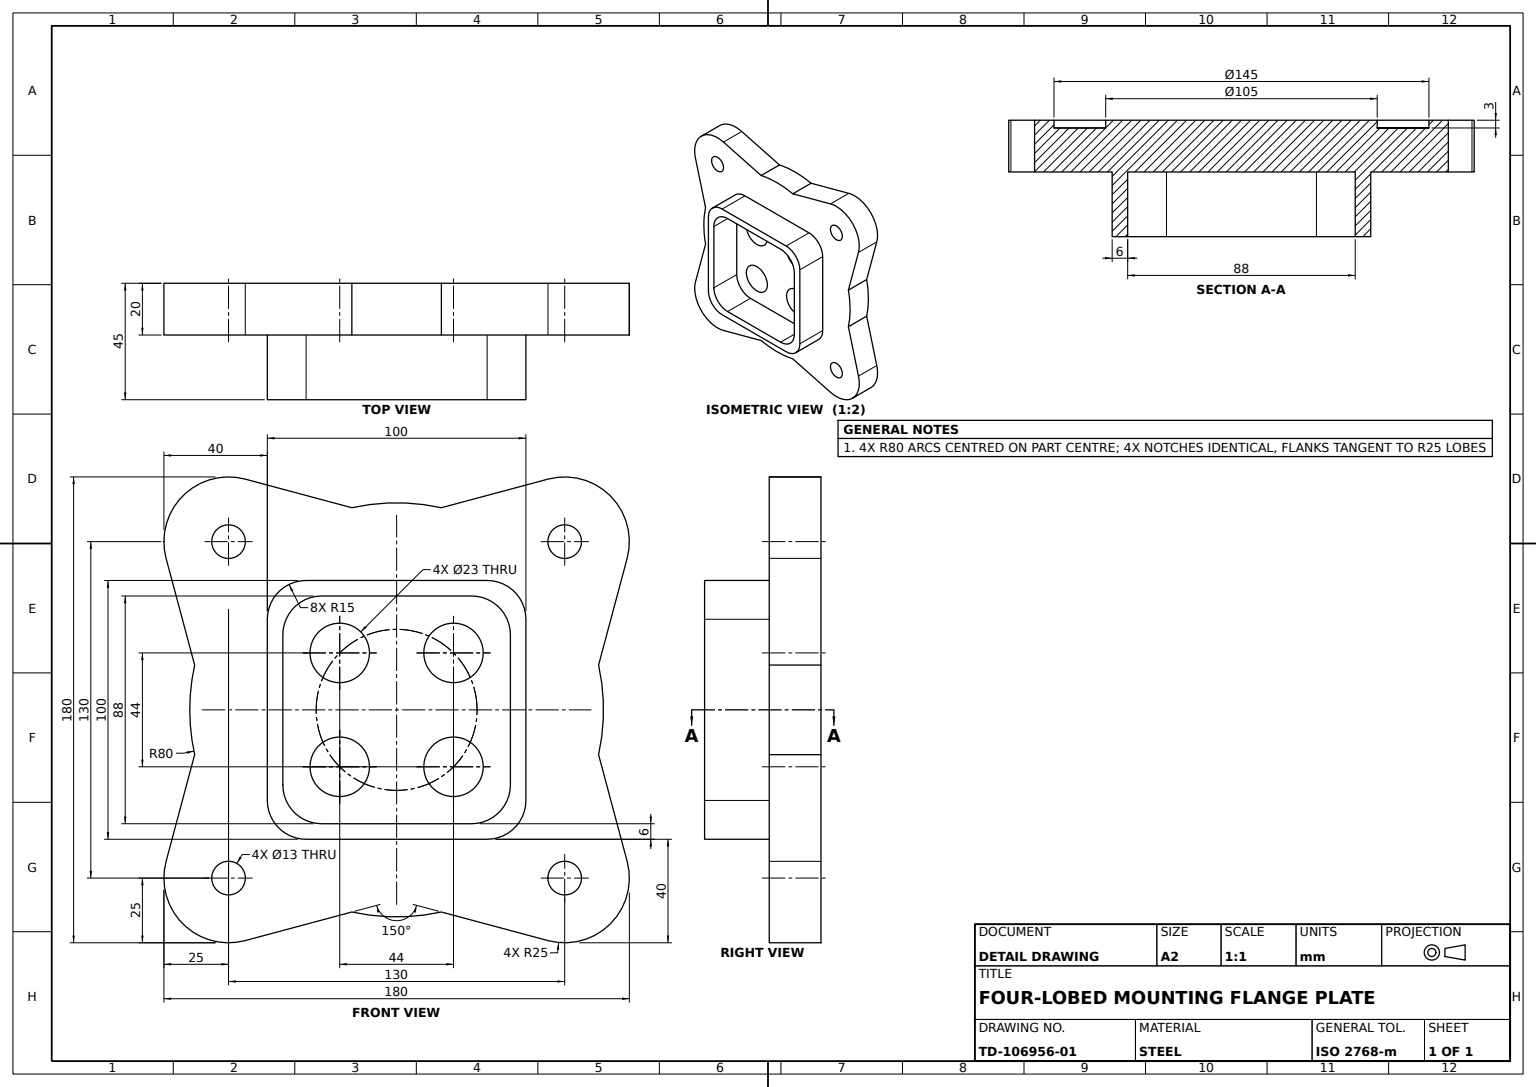
solid
v1 (89.148146,-58.529524,20)
v2 (89.148146,-58.529524,0)
e1 v1 v2 LINE
v3 (78.104184,-17.312898,0)
e2 v2 v3 LINE
v4 (78.104184,-17.312898,20)
e3 v4 v3 LINE
e4 v1 v4 LINE
face PLANE(AX(P(68.543971,18.366302,20),D(-0.965925826,-0.258819045,0),D(0.258819045,-0.965925826,0))) rev [e1 e2 -e3 -e4]
v5 (52.5,0,3)
v6 (-52.5,0,3)
e5 v5 v6 CIRCLE(AX(P(0,0,3),D(0,0,-1),D(-1,0,0)),52.5)
v7 (-52.5,0,0)
e6 v6 v7 LINE
v8 (52.5,0,0)
e7 v8 v7 CIRCLE(AX(P(0,0,0),D(0,0,-1),D(-1,0,0)),52.5)
e8 v5 v8 LINE
face CYL(AX(P(0,0,3),D(0,0,-1),D(-1,0,0)),52.5) [e5 e6 -e7 -e8]
v9 (-50,35,45)
v10 (-35,50,45)
e9 v9 v10 CIRCLE(AX(P(-35,35,45),D(0,0,-1),D(1,0,0)),15)
v11 (-35,50,20)
e10 v10 v11 LINE
v12 (-50,35,20)
e11 v12 v11 CIRCLE(AX(P(-35,35,20),D(0,0,-1),D(1,0,0)),15)
e12 v9 v12 LINE
face CYL(AX(P(-35,35,45),D(0,0,-1),D(-1,0,0)),15) [e9 e10 -e11 -e12]
e13 v6 v5 CIRCLE(AX(P(0,0,3),D(0,0,-1),D(-1,0,0)),52.5)
v13 (-72.5,0,3)
v14 (72.5,0,3)
e14 v13 v14 CIRCLE(AX(P(0,0,3),D(0,0,-1),D(-1,0,0)),72.5)
e15 v14 v13 CIRCLE(AX(P(0,0,3),D(0,0,-1),D(-1,0,0)),72.5)
face PLANE(AX(P(0,0,3),D(0,0,-1),D(-1,0,0))) [-e5 -e13] [e14 e15]
v15 (-50,-35,45)
e16 v15 v9 LINE
v16 (-35,-50,45)
e17 v15 v16 CIRCLE(AX(P(-35,-35,45),D(0,0,1),D(1,0,0)),15)
v17 (35,-50,45)
e18 v16 v17 LINE
v18 (50,-35,45)
e19 v17 v18 CIRCLE(AX(P(35,-35,45),D(0,0,1),D(1,0,0)),15)
v19 (50,35,45)
e20 v18 v19 LINE
v20 (35,50,45)
e21 v19 v20 CIRCLE(AX(P(35,35,45),D(0,0,1),D(1,0,0)),15)
e22 v10 v20 LINE
v21 (-29,44,45)
v22 (29,44,45)
e23 v21 v22 LINE
v23 (44,29,45)
e24 v23 v22 CIRCLE(AX(P(29,29,45),D(0,0,1),D(1,0,0)),15)
v24 (44,-29,45)
e25 v24 v23 LINE
v25 (29,-44,45)
e26 v25 v24 CIRCLE(AX(P(29,-29,45),D(0,0,1),D(1,0,0)),15)
v26 (-29,-44,45)
e27 v26 v25 LINE
v27 (-44,-29,45)
e28 v26 v27 CIRCLE(AX(P(-29,-29,45),D(0,0,-1),D(1,0,0)),15)
v28 (-44,29,45)
e29 v27 v28 LINE
e30 v28 v21 CIRCLE(AX(P(-29,29,45),D(0,0,-1),D(1,0,0)),15)
face PLANE(AX(P(0,0,45),D(0,0,1),D(1,0,0))) [-e9 -e16 e17 e18 e19 e20 e21 -e22] [e23 -e24 -e25 -e26 -e27 e28 e29 e30]
v29 (-35,-50,20)
e31 v16 v29 LINE
v30 (-50,-35,20)
e32 v15 v30 LINE
e33 v30 v29 CIRCLE(AX(P(-35,-35,20),D(0,0,1),D(1,0,0)),15)
face CYL(AX(P(-35,-35,45),D(0,0,-1),D(-1,0,0)),15) [-e31 -e17 e32 e33]
v31 (78.104184,17.312898,20)
e34 v4 v31 CIRCLE(AX(P(0,0,20),D(0,0,1),D(1,0,0)),80)
v32 (78.104184,17.312898,0)
e35 v3 v32 CIRCLE(AX(P(0,0,0),D(0,0,1),D(1,0,0)),80)
e36 v31 v32 LINE
face CYL(AX(P(0,0,20),D(0,0,-1),D(-1,0,0)),80) [-e34 e3 e35 -e36]
v33 (-10.5,22,20)
v34 (-10.5,22,0)
e37 v33 v34 LINE
v35 (-33.5,22,0)
e38 v35 v34 CIRCLE(AX(P(-22,22,0),D(0,0,1),D(1,0,0)),11.5)
v36 (-33.5,22,20)
e39 v36 v35 LINE
e40 v36 v33 CIRCLE(AX(P(-22,22,20),D(0,0,1),D(1,0,0)),11.5)
face CYL(AX(P(-22,22,20),D(0,0,-1),D(-1,0,0)),11.5) rev [e37 -e38 -e39 e40]
v37 (-58.529528,89.148147,0)
v38 (-90,65,0)
e41 v37 v38 CIRCLE(AX(P(-65,65,0),D(0,0,1),D(1,0,0)),25)
v39 (-90,65,20)
e42 v39 v38 LINE
v40 (-58.529528,89.148147,20)
e43 v40 v39 CIRCLE(AX(P(-65,65,20),D(0,0,1),D(1,0,0)),25)
e44 v40 v37 LINE
face CYL(AX(P(-65,65,20),D(0,0,-1),D(-1,0,0)),25) [e41 -e42 -e43 e44]
v41 (-58.529528,-89.148147,0)
v42 (-17.312898,-78.104184,0)
e45 v41 v42 LINE
v43 (-17.312898,-78.104184,20)
e46 v43 v42 LINE
v44 (-58.529528,-89.148147,20)
e47 v44 v43 LINE
e48 v44 v41 LINE
face PLANE(AX(P(18.366302,-68.543971,20),D(-0.258819045,0.965925826,0),D(-0.965925826,-0.258819045,0))) rev [e45 -e46 -e47 e48]
v45 (50,35,20)
e49 v19 v45 LINE
v46 (35,50,20)
e50 v45 v46 CIRCLE(AX(P(35,35,20),D(0,0,1),D(1,0,0)),15)
e51 v20 v46 LINE
face CYL(AX(P(35,35,45),D(0,0,-1),D(-1,0,0)),15) [e49 e50 -e51 -e21]
v47 (-80,0,20)
v48 (-80,0,0)
e52 v47 v48 LINE
v49 (-78.104184,17.312898,20)
e53 v49 v47 CIRCLE(AX(P(0,0,20),D(0,0,1),D(1,0,0)),80)
v50 (-78.104184,17.312898,0)
e54 v49 v50 LINE
e55 v50 v48 CIRCLE(AX(P(0,0,0),D(0,0,1),D(1,0,0)),80)
face CYL(AX(P(0,0,20),D(0,0,-1),D(-1,0,0)),80) [-e52 -e53 e54 e55]
v51 (-44,-29,20)
e56 v27 v51 LINE
v52 (-44,29,20)
e57 v51 v52 LINE
e58 v28 v52 LINE
face PLANE(AX(P(-44,0,45),D(-1,0,0),D(0,0,1))) rev [-e29 e56 e57 -e58]
v53 (-72.5,0,0)
v54 (72.5,0,0)
e59 v53 v54 CIRCLE(AX(P(0,0,0),D(0,0,-1),D(-1,0,0)),72.5)
e60 v54 v53 CIRCLE(AX(P(0,0,0),D(0,0,-1),D(-1,0,0)),72.5)
v55 (-58.5,-65,0)
v56 (-71.5,-65,0)
e61 v55 v56 CIRCLE(AX(P(-65,-65,0),D(0,0,1),D(1,0,0)),6.5)
e62 v56 v55 CIRCLE(AX(P(-65,-65,0),D(0,0,1),D(1,0,0)),6.5)
v57 (-71.5,65,0)
v58 (-58.5,65,0)
e63 v57 v58 CIRCLE(AX(P(-65,65,0),D(0,0,1),D(1,0,0)),6.5)
e64 v58 v57 CIRCLE(AX(P(-65,65,0),D(0,0,1),D(1,0,0)),6.5)
v59 (58.500003,-65.000003,0)
v60 (71.500003,-65.000003,0)
e65 v59 v60 CIRCLE(AX(P(65.000003,-65.000003,0),D(0,0,1),D(1,0,0)),6.5)
e66 v60 v59 CIRCLE(AX(P(65.000003,-65.000003,0),D(0,0,1),D(1,0,0)),6.5)
v61 (-90,-65,0)
e67 v61 v41 CIRCLE(AX(P(-65,-65,0),D(0,0,1),D(1,0,0)),25)
v62 (-89.148146,-58.529524,0)
e68 v62 v61 CIRCLE(AX(P(-65,-65,0),D(0,0,1),D(1,0,0)),25)
v63 (-78.104184,-17.312898,0)
e69 v62 v63 LINE
e70 v48 v63 CIRCLE(AX(P(0,0,0),D(0,0,1),D(1,0,0)),80)
v64 (-89.148146,58.529524,0)
e71 v64 v50 LINE
e72 v38 v64 CIRCLE(AX(P(-65,65,0),D(0,0,1),D(1,0,0)),25)
v65 (-17.312881,78.104188,0)
e73 v37 v65 LINE
v66 (17.312898,78.104184,0)
e74 v66 v65 CIRCLE(AX(P(0,0,0),D(0,0,1),D(1,0,0)),80)
v67 (58.529528,89.148147,0)
e75 v67 v66 LINE
v68 (89.148146,58.529524,0)
e76 v68 v67 CIRCLE(AX(P(64.999998,64.999998,0),D(0,0,1),D(1,0,0)),25.000001)
e77 v68 v32 LINE
v69 (58.529528,-89.148147,0)
e78 v69 v2 CIRCLE(AX(P(65.000003,-65.000003,0),D(0,0,1),D(1,0,0)),24.999998)
v70 (17.312881,-78.104188,0)
e79 v69 v70 LINE
e80 v42 v70 CIRCLE(AX(P(0,0,0),D(0,0,1),D(1,0,0)),80)
v71 (71.499998,64.999998,0)
v72 (58.499998,64.999998,0)
e81 v71 v72 CIRCLE(AX(P(64.999998,64.999998,0),D(0,0,1),D(1,0,0)),6.5)
e82 v72 v71 CIRCLE(AX(P(64.999998,64.999998,0),D(0,0,1),D(1,0,0)),6.5)
face PLANE(AX(P(0,0,0),D(0,0,1),D(1,0,0))) rev [-e59 -e60] [e61 e62] [e63 e64] [e65 e66] [-e67 -e68 e69 -e70 -e55 -e71 -e72 -e41 e73 -e74 -e75 -e76 e77 -e35 -e2 -e78 e79 -e80 -e45] [e81 e82]
v73 (58.500003,-65.000003,20)
e83 v73 v59 LINE
v74 (71.500003,-65.000003,20)
e84 v73 v74 CIRCLE(AX(P(65.000003,-65.000003,20),D(0,0,1),D(1,0,0)),6.5)
e85 v74 v60 LINE
face CYL(AX(P(65.000003,-65.000003,20),D(0,0,-1),D(-1,0,0)),6.5) rev [-e65 -e83 e84 e85]
v75 (58.529528,-89.148147,20)
e86 v75 v69 LINE
e87 v75 v1 CIRCLE(AX(P(65.000003,-65.000003,20),D(0,0,1),D(1,0,0)),24.999998)
face CYL(AX(P(65.000003,-65.000003,20),D(0,0,-1),D(-1,0,0)),24.999998) [e86 e78 -e1 -e87]
v76 (17.312898,78.104184,20)
e88 v76 v66 LINE
v77 (-17.312881,78.104188,20)
e89 v77 v65 LINE
e90 v76 v77 CIRCLE(AX(P(0,0,20),D(0,0,1),D(1,0,0)),80)
face CYL(AX(P(0,0,20),D(0,0,-1),D(-1,0,0)),80) [e88 e74 -e89 -e90]
v78 (-90,-65,20)
e91 v78 v61 LINE
v79 (-89.148146,-58.529524,20)
e92 v79 v78 CIRCLE(AX(P(-65,-65,20),D(0,0,1),D(1,0,0)),25)
e93 v79 v62 LINE
face CYL(AX(P(-65,-65,20),D(0,0,-1),D(-1,0,0)),25) [-e91 -e92 e93 e68]
e94 v40 v77 LINE
face PLANE(AX(P(18.366293,68.543989,20),D(0.258818868,0.965925874,0),D(-0.965925874,0.258818868,0))) [-e44 e94 e89 -e73]
v80 (89.148146,58.529524,20)
e95 v80 v68 LINE
e96 v80 v31 LINE
face PLANE(AX(P(68.543971,-18.366302,20),D(0.965925826,-0.258819045,0),D(0.258819045,0.965925826,0))) [-e77 -e95 e96 e36]
e97 v74 v73 CIRCLE(AX(P(65.000003,-65.000003,20),D(0,0,1),D(1,0,0)),6.5)
face CYL(AX(P(65.000003,-65.000003,20),D(0,0,-1),D(-1,0,0)),6.5) rev [-e66 -e85 e97 e83]
v81 (50,-35,20)
e98 v18 v81 LINE
e99 v81 v45 LINE
face PLANE(AX(P(50,0,45),D(-1,0,0),D(0,0,1))) rev [e98 e99 -e49 -e20]
v82 (-58.5,-65,20)
e100 v82 v55 LINE
v83 (-71.5,-65,20)
e101 v82 v83 CIRCLE(AX(P(-65,-65,20),D(0,0,1),D(1,0,0)),6.5)
e102 v83 v56 LINE
face CYL(AX(P(-65,-65,20),D(0,0,-1),D(-1,0,0)),6.5) rev [-e61 -e100 e101 e102]
e103 v30 v12 LINE
face PLANE(AX(P(-50,0,45),D(-1,0,0),D(0,0,1))) [-e103 -e32 e16 e12]
v84 (58.529528,89.148147,20)
e104 v84 v67 LINE
e105 v84 v76 LINE
face PLANE(AX(P(-18.366302,68.543971,20),D(0.258819045,-0.965925826,0),D(0.965925826,0.258819045,0))) rev [e104 e75 -e88 -e105]
v85 (17.312881,-78.104188,20)
e106 v85 v70 LINE
e107 v43 v85 CIRCLE(AX(P(0,0,20),D(0,0,1),D(1,0,0)),80)
face CYL(AX(P(0,0,20),D(0,0,-1),D(-1,0,0)),80) [e80 -e106 -e107 e46]
v86 (-10.5,-22,20)
v87 (-10.5,-22,0)
e108 v86 v87 LINE
v88 (-33.5,-22,0)
e109 v88 v87 CIRCLE(AX(P(-22,-22,0),D(0,0,1),D(1,0,0)),11.5)
v89 (-33.5,-22,20)
e110 v89 v88 LINE
e111 v89 v86 CIRCLE(AX(P(-22,-22,20),D(0,0,1),D(1,0,0)),11.5)
face CYL(AX(P(-22,-22,20),D(0,0,-1),D(-1,0,0)),11.5) rev [e108 -e109 -e110 e111]
v90 (-29,-44,20)
e112 v90 v51 CIRCLE(AX(P(-29,-29,20),D(0,0,-1),D(1,0,0)),15)
e113 v26 v90 LINE
face CYL(AX(P(-29,-29,45),D(0,0,-1),D(-1,0,0)),15) rev [e112 -e56 -e28 e113]
e114 v80 v84 CIRCLE(AX(P(64.999998,64.999998,20),D(0,0,1),D(1,0,0)),25.000001)
face CYL(AX(P(64.999998,64.999998,20),D(0,0,-1),D(-1,0,0)),25.000001) [e95 e76 -e104 -e114]
v91 (10.5,22,20)
v92 (10.5,22,0)
e115 v91 v92 LINE
v93 (33.5,22,0)
e116 v93 v92 CIRCLE(AX(P(22,22,0),D(0,0,1),D(1,0,0)),11.5)
v94 (33.5,22,20)
e117 v94 v93 LINE
e118 v94 v91 CIRCLE(AX(P(22,22,20),D(0,0,1),D(1,0,0)),11.5)
face CYL(AX(P(22,22,20),D(0,0,-1),D(-1,0,0)),11.5) rev [e115 -e116 -e117 e118]
v95 (44,29,20)
e119 v23 v95 LINE
v96 (29,44,20)
e120 v22 v96 LINE
e121 v95 v96 CIRCLE(AX(P(29,29,20),D(0,0,1),D(1,0,0)),15)
face CYL(AX(P(29,29,45),D(0,0,-1),D(-1,0,0)),15) rev [-e119 e24 e120 -e121]
v97 (-71.5,65,20)
v98 (-58.5,65,20)
e122 v97 v98 CIRCLE(AX(P(-65,65,20),D(0,0,1),D(1,0,0)),6.5)
e123 v98 v58 LINE
e124 v97 v57 LINE
face CYL(AX(P(-65,65,20),D(0,0,-1),D(-1,0,0)),6.5) rev [e122 e123 -e63 -e124]
v99 (44,-29,20)
e125 v99 v95 LINE
e126 v24 v99 LINE
face PLANE(AX(P(44,0,45),D(-1,0,0),D(0,0,1))) [e25 e119 -e125 -e126]
e127 v13 v53 LINE
e128 v14 v54 LINE
face CYL(AX(P(0,0,3),D(0,0,-1),D(-1,0,0)),72.5) rev [e127 e59 -e128 -e14]
v100 (-89.148146,58.529524,20)
e129 v100 v64 LINE
e130 v100 v49 LINE
face PLANE(AX(P(-68.543971,-18.366302,20),D(0.965925826,0.258819045,0),D(-0.258819045,0.965925826,0))) rev [e129 e71 -e54 -e130]
v101 (29,-44,20)
e131 v101 v99 CIRCLE(AX(P(29,-29,20),D(0,0,1),D(1,0,0)),15)
e132 v25 v101 LINE
face CYL(AX(P(29,-29,45),D(0,0,-1),D(-1,0,0)),15) rev [e26 e126 -e131 -e132]
e133 v7 v8 CIRCLE(AX(P(0,0,0),D(0,0,-1),D(-1,0,0)),52.5)
face CYL(AX(P(0,0,3),D(0,0,-1),D(-1,0,0)),52.5) [-e6 e13 e8 -e133]
v102 (10.5,-22,20)
v103 (10.5,-22,0)
e134 v102 v103 LINE
v104 (33.5,-22,20)
e135 v102 v104 CIRCLE(AX(P(22,-22,20),D(0,0,1),D(1,0,0)),11.5)
v105 (33.5,-22,0)
e136 v104 v105 LINE
e137 v103 v105 CIRCLE(AX(P(22,-22,0),D(0,0,1),D(1,0,0)),11.5)
face CYL(AX(P(22,-22,20),D(0,0,-1),D(-1,0,0)),11.5) rev [-e134 e135 e136 -e137]
v106 (-78.104184,-17.312898,20)
e138 v106 v63 LINE
e139 v47 v106 CIRCLE(AX(P(0,0,20),D(0,0,1),D(1,0,0)),80)
face CYL(AX(P(0,0,20),D(0,0,-1),D(-1,0,0)),80) [-e138 -e139 e52 e70]
e140 v104 v102 CIRCLE(AX(P(22,-22,20),D(0,0,1),D(1,0,0)),11.5)
e141 v105 v103 CIRCLE(AX(P(22,-22,0),D(0,0,1),D(1,0,0)),11.5)
face CYL(AX(P(22,-22,20),D(0,0,-1),D(-1,0,0)),11.5) rev [e140 e134 -e141 -e136]
e142 v75 v85 LINE
face PLANE(AX(P(-18.366293,-68.543989,20),D(-0.258818868,-0.965925874,0),D(0.965925874,-0.258818868,0))) [-e86 e142 e106 -e79]
e143 v34 v35 CIRCLE(AX(P(-22,22,0),D(0,0,1),D(1,0,0)),11.5)
e144 v33 v36 CIRCLE(AX(P(-22,22,20),D(0,0,1),D(1,0,0)),11.5)
face CYL(AX(P(-22,22,20),D(0,0,-1),D(-1,0,0)),11.5) rev [e39 -e143 -e37 e144]
v107 (35,-50,20)
e145 v17 v107 LINE
e146 v107 v81 CIRCLE(AX(P(35,-35,20),D(0,0,1),D(1,0,0)),15)
face CYL(AX(P(35,-35,45),D(0,0,-1),D(-1,0,0)),15) [-e19 e145 e146 -e98]
e147 v91 v94 CIRCLE(AX(P(22,22,20),D(0,0,1),D(1,0,0)),11.5)
v108 (-29,44,20)
e148 v108 v96 LINE
e149 v52 v108 CIRCLE(AX(P(-29,29,20),D(0,0,-1),D(1,0,0)),15)
e150 v90 v101 LINE
e151 v86 v89 CIRCLE(AX(P(-22,-22,20),D(0,0,1),D(1,0,0)),11.5)
face PLANE(AX(P(0,0,20),D(0,0,1),D(1,0,0))) [-e140 -e135] [-e118 -e147] [-e148 -e149 -e57 -e112 e150 e131 e125 e121] [-e151 -e111] [-e40 -e144]
e152 v29 v107 LINE
e153 v11 v46 LINE
v109 (71.499998,64.999998,20)
v110 (58.499998,64.999998,20)
e154 v109 v110 CIRCLE(AX(P(64.999998,64.999998,20),D(0,0,1),D(1,0,0)),6.5)
e155 v110 v109 CIRCLE(AX(P(64.999998,64.999998,20),D(0,0,1),D(1,0,0)),6.5)
e156 v39 v100 CIRCLE(AX(P(-65,65,20),D(0,0,1),D(1,0,0)),25)
e157 v79 v106 LINE
e158 v78 v44 CIRCLE(AX(P(-65,-65,20),D(0,0,1),D(1,0,0)),25)
e159 v83 v82 CIRCLE(AX(P(-65,-65,20),D(0,0,1),D(1,0,0)),6.5)
e160 v98 v97 CIRCLE(AX(P(-65,65,20),D(0,0,1),D(1,0,0)),6.5)
face PLANE(AX(P(0,0,20),D(0,0,1),D(1,0,0))) [-e84 -e97] [-e152 -e33 e103 e11 e153 -e50 -e99 -e146] [-e154 -e155] [e34 -e96 e114 e105 e90 -e94 e43 e156 e130 e53 e139 -e157 e92 e158 e47 e107 -e142 e87 e4] [-e159 -e101] [-e122 -e160]
e161 v87 v88 CIRCLE(AX(P(-22,-22,0),D(0,0,1),D(1,0,0)),11.5)
face CYL(AX(P(-22,-22,20),D(0,0,-1),D(-1,0,0)),11.5) rev [-e161 -e108 e151 e110]
e162 v92 v93 CIRCLE(AX(P(22,22,0),D(0,0,1),D(1,0,0)),11.5)
face PLANE(AX(P(0,0,0),D(0,0,1),D(1,0,0))) rev [e162 e116] [e7 e133] [e141 e137] [e143 e38] [e161 e109]
e163 v21 v108 LINE
face PLANE(AX(P(0,44,45),D(0,1,0),D(0,0,1))) rev [-e120 -e23 e163 e148]
face CYL(AX(P(22,22,20),D(0,0,-1),D(-1,0,0)),11.5) rev [-e115 e147 e117 -e162]
e164 v110 v72 LINE
e165 v109 v71 LINE
face CYL(AX(P(64.999998,64.999998,20),D(0,0,-1),D(-1,0,0)),6.5) rev [e154 e164 -e81 -e165]
face CYL(AX(P(-65,65,20),D(0,0,-1),D(-1,0,0)),6.5) rev [e160 e124 -e64 -e123]
face CYL(AX(P(0,0,3),D(0,0,-1),D(-1,0,0)),72.5) rev [-e127 -e15 e128 e60]
face CYL(AX(P(-65,-65,20),D(0,0,-1),D(-1,0,0)),25) [e67 -e48 -e158 e91]
face PLANE(AX(P(0,-44,45),D(0,1,0),D(0,0,1))) [-e113 e27 e132 -e150]
face PLANE(AX(P(0,-50,45),D(0,1,0),D(0,0,1))) rev [e152 -e145 -e18 e31]
face CYL(AX(P(-65,-65,20),D(0,0,-1),D(-1,0,0)),6.5) rev [e100 -e62 -e102 e159]
face CYL(AX(P(64.999998,64.999998,20),D(0,0,-1),D(-1,0,0)),6.5) rev [-e164 e155 e165 -e82]
face PLANE(AX(P(0,50,45),D(0,1,0),D(0,0,1))) [-e10 e22 e51 -e153]
face PLANE(AX(P(-68.543971,18.366302,20),D(-0.965925826,0.258819045,0),D(-0.258819045,-0.965925826,0))) [-e69 -e93 e157 e138]
face CYL(AX(P(-29,29,45),D(0,0,-1),D(-1,0,0)),15) rev [-e163 -e30 e58 e149]
face CYL(AX(P(-65,65,20),D(0,0,-1),D(-1,0,0)),25) [-e129 -e156 e42 e72]
